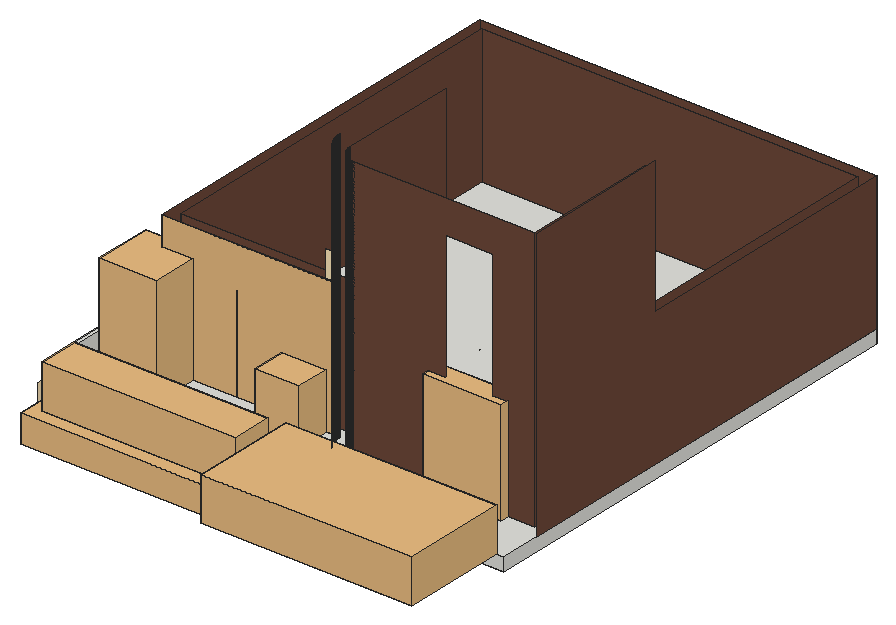
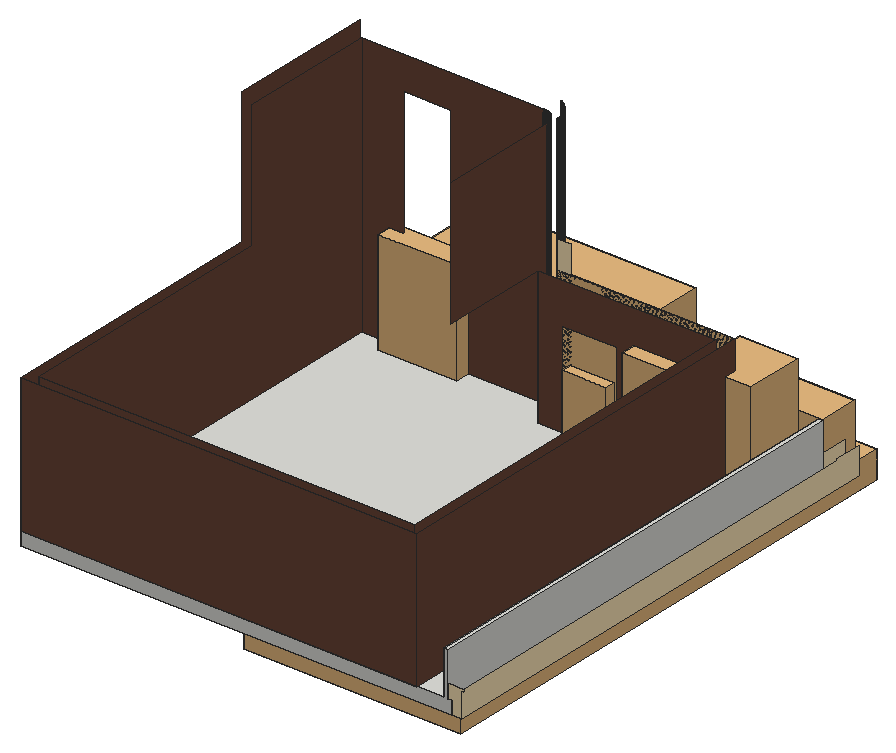
# SketchUp Ruby script. Lengths in inches.
U = 1.inch
M = Sketchup.active_model
def pt(a) = Geom::Point3d.new(a.map { |v| v * U })
def face(e, loops, mat)
  f = e.add_face(loops[0].map { |a| pt(a) })
  loops[1..].each { |l| e.add_face(l.map { |a| pt(a) }).erase! }
  f.material = f.back_material = mat if mat
  f
end
# faces: each face lists its corners as indices into pts; further lists are holes
def faces(e, pts, list, mat = nil) = list.each { |f| face(e, (f[0].is_a?(Array) ? f : [f]).map { |l| l.map { |i| pts[i] } }, mat) }
# xy, xz, yz: faces in a plane at the given z, y or x. An outline is a flat list of corners, or four numbers for a rectangle; further outlines are holes
def ring(l) = l.size == 4 ? [[l[0], l[1]], [l[2], l[1]], [l[2], l[3]], [l[0], l[3]]] : l.each_slice(2).to_a
def flat(e, list, mat, &to3) = list.each { |f| face(e, (f[0].is_a?(Array) ? f : [f]).map { |l| ring(l).map { |u, v| to3.(u, v) } }, mat) }
def xy(e, z, list, mat = nil) = flat(e, list, mat) { |x, y| [x, y, z] }
def xz(e, y, list, mat = nil) = flat(e, list, mat) { |x, z| [x, y, z] }
def yz(e, x, list, mat = nil) = flat(e, list, mat) { |y, z| [x, y, z] }
def lines(e, pts, list) = list.each { |a, b| e.add_line(pt(pts[a]), pt(pts[b])) }
# prism: a flat outline (further loops are holes) pulled along v
def prism(e, loops, v, mat = nil)
  f = face(e, loops, mat); d = Geom::Vector3d.new(v.map { |x| x * U })
  f.pushpull(f.normal.samedirection?(d) ? d.length : -d.length)
end
def box(e, o, s, mat = nil) = prism(e, [[o, [o[0] + s[0], o[1], o[2]], [o[0] + s[0], o[1] + s[1], o[2]], [o[0], o[1] + s[1], o[2]]]], [0, 0, s[2]], mat)
def at(x, y, z, deg = 0) = Geom::Transformation.translation(pt([x, y, z])) * Geom::Transformation.rotation(ORIGIN, Z_AXIS, deg.degrees)
def axes(o, x, y, z) = Geom::Transformation.new([*x, 0, *y, 0, *z, 0, *pt(o).to_a, 1])
def part(name) = M.definitions.add(name)
# library, detail: a bought-in or finely detailed component or shape, given as its bounding box
def library(name, o, s) = part(name).tap { |d| box(d.entities, o, s) }
def detail(e, o, s) = box(e.add_group.entities, o, s)
def put(e, d, t, mat = nil) = e.add_instance(d, t).tap { |i| i.material = mat if mat }
def group(e, t, mat = nil) = e.add_group.tap { |g| g.transformation = t; g.material = mat if mat }.entities
root = M.entities
M.materials.add("1026 AP 7946 SUNNY SIDE UP").color = [254, 231, 186]
M.materials.add("1916 AP K226 Macadamia Cream-N").color = [109, 72, 58]
M.materials.add("[Steel Brushed Stainless]").color = [48, 48, 48]
M.materials.add("[Wood Cherry Original]").color = [152, 86, 42]
c1 = library("Group\#76",[0,0,0],[126.13,128.06,238.18])
c2 = library("12",[-59.59,-13.96,-2.03],[132.77,19.46,130.2])
c3 = library("plant",[-35.72,-28.42,0],[66.31,67.39,84.38])
c4 = library("Group\#41",[0,-0.25,0],[156,0.25,120])
c5 = library("Glass Door",[0,0,0],[72,3.54,96])
c6 = library("Group\#22",[0,0,0],[186.93,93,38])
c7 = library("Group\#29",[0,0,0],[170,35.5,38])
c8 = library("Group\#53",[0,0,0.49],[191,455,12.72])
xy(root,132,[[15.03,254,18,674]],"1026 AP 7946 SUNNY SIDE UP")
xy(root,132,[[384,302,384,665,54,665,54,335,69,335,69,326,45,326,45,674,393,674,393,302],[224.53,302,224.29,302.01,224.06,302.02,223.82,302.03,223.59,302.04,223.35,302.06,223.12,302.07,222.88,302.09,222.65,302.12,222.41,302.14,221.95,302.2,221.71,302.23,221.48,302.26,221.25,302.3,221.01,302.33,220.55,302.42,220.32,302.46,219.86,302.56,219.625,302.61,219.4,302.66,218.71,302.84,218.49,302.9,218.26,302.97,218.03,303.03,217.81,303.1,217.58,303.17,217.36,303.25,217.14,303.32,216.91,303.4,216.69,303.48,216.47,303.57,216.25,303.65,216.03,303.74,215.82,303.83,215.38,304.01,215.17,304.11,214.95,304.2,214.74,304.3,214.53,304.41,214.31,304.51,214.1,304.62,213.89,304.72,213.6875,304.83,213.48,304.95,213.27,305.06,213.07,305.18,212.86,305.29,212.66,305.41,212.46,305.54,212.26,305.66,212.0625,305.79,211.86,305.91,211.67,306.04,211.47,306.18,211.28,306.31,211.08,306.45,210.89,306.58,210.51,306.86,210.33,307.01,210.14,307.15,209.96,307.3,209.77,307.45,209.23,307.9,209.06,308.06,208.88,308.22,208.71,308.375,208.54,308.54,208.2,308.86,207.86,309.2,207.54,309.54,207.375,309.71,207.22,309.88,207.06,310.06,206.9,310.23,206.45,310.77,206.3,310.96,206.15,311.14,206.01,311.33,205.86,311.51,205.58,311.89,205.45,312.08,205.31,312.28,205.18,312.47,205.04,312.67,204.91,312.86,204.79,313.0625,204.66,313.26,204.54,313.46,204.41,313.66,204.29,313.86,204.18,314.07,204.06,314.27,203.95,314.48,203.83,314.6875,203.72,314.89,203.62,315.1,203.51,315.31,203.41,315.53,203.3,315.74,203.2,315.95,203.11,316.17,203.01,316.38,202.83,316.82,202.74,317.03,202.65,317.25,202.57,317.47,202.48,317.69,202.4,317.91,202.32,318.14,202.25,318.36,202.17,318.58,202.1,318.81,202.03,319.03,201.97,319.26,201.9,319.49,201.84,319.71,201.66,320.4,201.61,320.625,201.56,320.86,201.46,321.32,201.42,321.55,201.33,322.01,201.3,322.25,201.26,322.48,201.23,322.71,201.2,322.95,201.14,323.41,201.12,323.65,201.09,323.88,201.07,324.12,201.06,324.35,201.04,324.59,201.03,324.82,201.02,325.06,201.01,325.29,201,325.53,201,326,111,326,111,335,210,335,210,311,224.85,311,224.85,302],[311.52,302,347.52,311],[210,311,210,325.85,210,325.71,210.01,325.56,210.01,325.41,210.02,325.26,210.03,325.12,210.05,324.82,210.06,324.68,210.07,324.53,210.09,324.38,210.1,324.24,210.14,323.94,210.16,323.8,210.18,323.65,210.21,323.51,210.23,323.36,210.26,323.22,210.29,323.07,210.35,322.79,210.38,322.64,210.41,322.5,210.45,322.36,210.49,322.21,210.52,322.07,210.5625,321.93,210.6,321.79,210.65,321.65,210.6875,321.51,210.73,321.36,210.78,321.22,210.83,321.09,210.875,320.95,210.93,320.81,211.03,320.53,211.09,320.4,211.14,320.26,211.26,319.99,211.32,319.85,211.44,319.59,211.5,319.45,211.57,319.32,211.63,319.19,211.91,318.67,211.99,318.54,212.06,318.42,212.13,318.29,212.21,318.16,212.29,318.04,212.37,317.91,212.53,317.67,212.61,317.54,212.69,317.42,212.78,317.3,212.86,317.18,212.95,317.06,213.04,316.95,213.22,316.71,213.3125,316.6,213.4,316.48,213.5,316.37,213.59,316.26,214.09,315.71,214.1875,315.6,214.29,315.5,214.39,315.39,214.5,315.29,214.6,315.1875,214.71,315.09,215.26,314.59,215.37,314.5,215.48,314.4,215.6,314.3125,215.71,314.22,215.95,314.04,216.06,313.95,216.18,313.86,216.3,313.78,216.42,313.69,216.54,313.61,216.67,313.53,216.91,313.37,217.04,313.29,217.16,313.21,217.29,313.13,217.42,313.06,217.54,312.99,217.67,312.91,218.19,312.63,218.32,312.57,218.45,312.5,218.59,312.44,218.85,312.32,218.99,312.26,219.26,312.14,219.4,312.09,219.53,312.03,219.81,311.93,219.95,311.875,220.09,311.83,220.22,311.78,220.36,311.73,220.51,311.6875,220.65,311.65,220.79,311.6,220.93,311.5625,221.07,311.52,221.21,311.49,221.36,311.45,221.5,311.41,221.64,311.38,221.79,311.35,222.07,311.29,222.22,311.26,222.36,311.23,222.51,311.21,222.65,311.18,222.8,311.16,222.94,311.14,223.24,311.1,223.38,311.09,223.53,311.07,223.68,311.06,223.82,311.05,224.12,311.03,224.26,311.02,224.41,311.01,224.56,311.01,224.71,311,224.85,311]],"1916 AP K226 Macadamia Cream-N")
xz(root,311,[[224.71,132,224.85,363],[[224.85,132,384,363],[305.52,138,347.52,333.89]]],"1916 AP K226 Macadamia Cream-N")
xz(root,311.01,[[224.41,132,224.56,363]],"1916 AP K226 Macadamia Cream-N")
xz(root,326,[[189,132,201,276]],"1026 AP 7946 SUNNY SIDE UP")
xz(root,326,[[[45,132,69,132,69,216,111,216,111,132,201,132,201,252,45,252],[141,162,189,216]]],"1916 AP K226 Macadamia Cream-N")
xz(root,335,[[[54,132,54,252,210,252,210,132,111,132,111,216,69,216,69,132],[141,162,189,216]]],"1916 AP K226 Macadamia Cream-N")
xz(root,665,[[54,132,384,252]],"1916 AP K226 Macadamia Cream-N")
xz(root,672,[[8,120,15,126]],"1026 AP 7946 SUNNY SIDE UP")
xz(root,674,[[6,120,6,142,4,142,4,144,18,144,18,132,15.03,132,15.03,126,15,126,15,120]],"1026 AP 7946 SUNNY SIDE UP")
xz(root,674,[[45,132,393,252]],"1916 AP K226 Macadamia Cream-N")
yz(root,6,[[239,120,239,144,262.9375,144,262.9375,142,674,142,674,120]],"1026 AP 7946 SUNNY SIDE UP")
yz(root,8,[[238.99,120,672,126]],"1026 AP 7946 SUNNY SIDE UP")
yz(root,15,[[672,120,674,126]],"1026 AP 7946 SUNNY SIDE UP")
yz(root,15.03,[[254,126,674,132]],"1026 AP 7946 SUNNY SIDE UP")
yz(root,18,[[239.06,132,674,144]],"1026 AP 7946 SUNNY SIDE UP")
yz(root,45,[[326,132,674,252]],"1916 AP K226 Macadamia Cream-N")
yz(root,54,[[335,132,665,252]],"1916 AP K226 Macadamia Cream-N")
yz(root,69,[[326,132,335,216]],"1916 AP K226 Macadamia Cream-N")
yz(root,111,[[326,132,335,216]],"1916 AP K226 Macadamia Cream-N")
yz(root,201,[[325.53,132,325.76,370],[325.76,132,326,370]],"1916 AP K226 Macadamia Cream-N")
yz(root,210,[[325.71,132,325.85,363],[325.85,132,335,132,335,252,431,252,431,363,325.85,363]],"1916 AP K226 Macadamia Cream-N")
yz(root,210.01,[[325.41,132,325.56,363]],"1916 AP K226 Macadamia Cream-N")
yz(root,384,[[311,132,311,363,431,363,431,252,665,252,665,132]],"1916 AP K226 Macadamia Cream-N")
yz(root,393,[[302,132,674,132,674,252,431,252,431,370,302,370]],"1916 AP K226 Macadamia Cream-N")
p = [[215.17,304.11,132],[215.17,304.11,370],[214.95,304.2,370],[214.95,304.2,132],[214.74,304.3,370],[214.74,304.3,132],
  [214.53,304.41,370],[214.53,304.41,132],[214.31,304.51,370],[214.31,304.51,132],[214.1,304.62,370],[214.1,304.62,132],
  [213.89,304.72,370],[213.89,304.72,132],[213.6875,304.83,370],[213.6875,304.83,132],[213.48,304.95,370],[213.48,304.95,132],
  [213.27,305.06,370],[213.27,305.06,132],[213.07,305.18,370],[213.07,305.18,132],[212.86,305.29,370],[212.86,305.29,132],
  [212.66,305.41,370],[212.66,305.41,132],[212.46,305.54,370],[212.46,305.54,132],[212.26,305.66,370],[212.26,305.66,132],
  [212.0625,305.79,370],[212.0625,305.79,132],[211.86,305.91,370],[211.86,305.91,132],[211.67,306.04,370],[211.67,306.04,132],
  [211.47,306.18,370],[211.47,306.18,132],[211.28,306.31,370],[211.28,306.31,132],[211.08,306.45,370],[211.08,306.45,132],
  [210.89,306.58,370],[210.89,306.58,132],[210.7,306.72,370],[210.7,306.72,132],[210.51,306.86,370],[210.51,306.86,132],
  [210.33,307.01,370],[210.33,307.01,132],[210.14,307.15,370],[210.14,307.15,132],[209.96,307.3,370],[209.96,307.3,132],
  [209.77,307.45,370],[209.77,307.45,132],[209.59,307.6,370],[209.59,307.6,132],[209.41,307.75,370],[209.41,307.75,132],
  [209.23,307.9,370],[209.23,307.9,132],[209.06,308.06,370],[209.06,308.06,132],[208.88,308.22,370],[208.88,308.22,132],
  [208.71,308.375,370],[208.71,308.375,132],[208.54,308.54,370],[208.54,308.54,132],[208.37,308.7,370],[208.37,308.7,132],
  [208.2,308.86,370],[208.2,308.86,132],[208.03,309.03,370],[208.03,309.03,132],[207.86,309.2,370],[207.86,309.2,132],
  [207.7,309.37,370],[207.7,309.37,132],[207.54,309.54,370],[207.54,309.54,132],[207.375,309.71,370],[207.375,309.71,132],
  [207.22,309.88,370],[207.22,309.88,132],[207.06,310.06,370],[207.06,310.06,132],[206.9,310.23,370],[206.9,310.23,132],
  [206.75,310.41,370],[206.75,310.41,132],[206.6,310.59,370],[206.6,310.59,132],[206.45,310.77,370],[206.45,310.77,132],
  [206.3,310.96,370],[206.3,310.96,132],[206.15,311.14,370],[206.15,311.14,132],[223.68,311.06,132],[223.68,311.06,363],
  [223.82,311.05,363],[223.82,311.05,132],[223.97,311.04,363],[223.97,311.04,132],[224.12,311.03,363],[224.12,311.03,132],
  [224.26,311.02,363],[224.26,311.02,132],[224.41,311.01,363],[224.41,311.01,132],[224.56,311.01,132],[224.56,311.01,363],
  [224.71,311,363],[224.71,311,132],[206.01,311.33,370],[206.01,311.33,132],[222.8,311.16,132],[222.8,311.16,363],
  [222.94,311.14,363],[222.94,311.14,132],[223.09,311.12,363],[223.09,311.12,132],[223.24,311.1,363],[223.24,311.1,132],
  [223.38,311.09,363],[223.38,311.09,132],[223.53,311.07,363],[223.53,311.07,132],[222.22,311.26,132],[222.22,311.26,363],
  [222.36,311.23,363],[222.36,311.23,132],[222.51,311.21,363],[222.51,311.21,132],[222.65,311.18,363],[222.65,311.18,132],
  [205.86,311.51,370],[205.86,311.51,132],[221.64,311.38,132],[221.64,311.38,363],[221.79,311.35,363],[221.79,311.35,132],
  [221.93,311.32,363],[221.93,311.32,132],[222.07,311.29,363],[222.07,311.29,132],[221.21,311.49,132],[221.21,311.49,363],
  [221.36,311.45,363],[221.36,311.45,132],[221.5,311.41,363],[221.5,311.41,132],[205.72,311.7,370],[205.72,311.7,132],
  [220.93,311.5625,132],[220.93,311.5625,363],[221.07,311.52,363],[221.07,311.52,132],[220.51,311.6875,132],[220.51,311.6875,363],
  [220.65,311.65,363],[220.65,311.65,132],[220.79,311.6,363],[220.79,311.6,132],[205.58,311.89,370],[205.58,311.89,132],
  [220.22,311.78,132],[220.22,311.78,363],[220.36,311.73,363],[220.36,311.73,132],[219.95,311.875,132],[219.95,311.875,363],
  [220.09,311.83,363],[220.09,311.83,132],[205.45,312.08,370],[205.45,312.08,132],[219.67,311.98,132],[219.67,311.98,363],
  [219.81,311.93,363],[219.81,311.93,132],[219.4,312.09,132],[219.4,312.09,363],[219.53,312.03,363],[219.53,312.03,132],
  [205.31,312.28,370],[205.31,312.28,132],[219.125,312.2,132],[219.125,312.2,363],[219.26,312.14,363],[219.26,312.14,132],
  [218.99,312.26,132],[218.99,312.26,363],[205.18,312.47,370],[205.18,312.47,132],[218.72,312.38,132],[218.72,312.38,363],
  [218.85,312.32,363],[218.85,312.32,132],[218.45,312.5,132],[218.45,312.5,363],[218.59,312.44,363],[218.59,312.44,132],
  [205.04,312.67,370],[205.04,312.67,132],[218.32,312.57,132],[218.32,312.57,363],[218.06,312.7,132],[218.06,312.7,363],
  [218.19,312.63,363],[218.19,312.63,132],[204.91,312.86,370],[204.91,312.86,132],[217.93,312.77,132],[217.93,312.77,363],
  [217.67,312.91,132],[217.67,312.91,363],[217.8,312.84,363],[217.8,312.84,132],[204.79,313.0625,370],[204.79,313.0625,132],
  [217.54,312.99,132],[217.54,312.99,363],[217.42,313.06,132],[217.42,313.06,363],[204.66,313.26,370],[204.66,313.26,132],
  [217.16,313.21,132],[217.16,313.21,363],[217.29,313.13,363],[217.29,313.13,132],[217.04,313.29,132],[217.04,313.29,363],
  [204.54,313.46,370],[204.54,313.46,132],[216.91,313.37,132],[216.91,313.37,363],[216.67,313.53,132],[216.67,313.53,363],
  [216.79,313.45,363],[216.79,313.45,132],[204.41,313.66,370],[204.41,313.66,132],[216.54,313.61,132],[216.54,313.61,363],
  [216.42,313.69,132],[216.42,313.69,363],[204.29,313.86,370],[204.29,313.86,132],[216.3,313.78,132],[216.3,313.78,363],
  [216.18,313.86,132],[216.18,313.86,363],[204.18,314.07,370],[204.18,314.07,132],[216.06,313.95,132],[216.06,313.95,363],
  [215.83,314.13,132],[215.83,314.13,363],[215.95,314.04,363],[215.95,314.04,132],[204.06,314.27,370],[204.06,314.27,132],
  [215.71,314.22,132],[215.71,314.22,363],[215.6,314.3125,132],[215.6,314.3125,363],[203.95,314.48,370],[203.95,314.48,132],
  [215.48,314.4,132],[215.48,314.4,363],[215.37,314.5,132],[215.37,314.5,363],[203.83,314.6875,370],[203.83,314.6875,132],
  [215.26,314.59,132],[215.26,314.59,363],[215.15,314.69,132],[215.15,314.69,363],[203.72,314.89,370],[203.72,314.89,132],
  [215.04,314.79,132],[215.04,314.79,363],[214.93,314.89,132],[214.93,314.89,363],[203.62,315.1,370],[203.62,315.1,132],
  [214.82,314.99,132],[214.82,314.99,363],[214.71,315.09,132],[214.71,315.09,363],[203.51,315.31,370],[203.51,315.31,132],
  [214.6,315.1875,132],[214.6,315.1875,363],[214.5,315.29,132],[214.5,315.29,363],[203.41,315.53,370],[203.41,315.53,132],
  [214.39,315.39,132],[214.39,315.39,363],[214.29,315.5,132],[214.29,315.5,363],[203.3,315.74,370],[203.3,315.74,132],
  [214.1875,315.6,132],[214.1875,315.6,363],[214.09,315.71,132],[214.09,315.71,363],[203.2,315.95,370],[203.2,315.95,132],
  [213.99,315.82,132],[213.99,315.82,363],[213.89,315.93,132],[213.89,315.93,363],[213.79,316.04,132],[213.79,316.04,363],
  [203.11,316.17,370],[203.11,316.17,132],[213.69,316.15,132],[213.69,316.15,363],[213.59,316.26,132],[213.59,316.26,363],
  [203.01,316.38,370],[203.01,316.38,132],[213.5,316.37,132],[213.5,316.37,363],[202.92,316.6,370],[202.92,316.6,132],
  [213.4,316.48,132],[213.4,316.48,363],[213.3125,316.6,132],[213.3125,316.6,363],[202.83,316.82,370],[202.83,316.82,132],
  [213.22,316.71,132],[213.22,316.71,363],[213.13,316.83,132],[213.13,316.83,363],[202.74,317.03,370],[202.74,317.03,132],
  [213.04,316.95,132],[213.04,316.95,363],[212.95,317.06,132],[212.95,317.06,363],[202.65,317.25,370],[202.65,317.25,132],
  [212.86,317.18,132],[212.86,317.18,363],[212.78,317.3,132],[212.78,317.3,363],[202.57,317.47,370],[202.57,317.47,132],
  [212.69,317.42,132],[212.69,317.42,363],[212.61,317.54,132],[212.61,317.54,363],[202.48,317.69,370],[202.48,317.69,132],
  [212.53,317.67,132],[212.53,317.67,363],[202.4,317.91,370],[202.4,317.91,132],[212.45,317.79,132],[212.45,317.79,363],
  [212.37,317.91,132],[212.37,317.91,363],[202.32,318.14,370],[202.32,318.14,132],[212.29,318.04,132],[212.29,318.04,363],
  [212.21,318.16,132],[212.21,318.16,363],[202.25,318.36,370],[202.25,318.36,132],[212.13,318.29,132],[212.13,318.29,363],
  [212.06,318.42,132],[212.06,318.42,363],[202.17,318.58,370],[202.17,318.58,132],[211.99,318.54,132],[211.99,318.54,363],
  [211.91,318.67,132],[211.91,318.67,363],[202.1,318.81,370],[202.1,318.81,132],[211.84,318.8,132],[211.84,318.8,363],
  [202.03,319.03,370],[202.03,319.03,132],[211.77,318.93,132],[211.77,318.93,363],[211.7,319.06,132],[211.7,319.06,363],
  [201.97,319.26,370],[201.97,319.26,132],[211.63,319.19,132],[211.63,319.19,363],[211.57,319.32,132],[211.57,319.32,363],
  [201.9,319.49,370],[201.9,319.49,132],[211.5,319.45,132],[211.5,319.45,363],[201.84,319.71,370],[201.84,319.71,132],
  [211.44,319.59,132],[211.44,319.59,363],[211.38,319.72,132],[211.38,319.72,363],[201.78,319.94,370],[201.78,319.94,132],
  [211.32,319.85,132],[211.32,319.85,363],[201.72,320.17,370],[201.72,320.17,132],[211.26,319.99,132],[211.26,319.99,363],
  [211.2,320.125,132],[211.2,320.125,363],[211.14,320.26,132],[211.14,320.26,363],[201.66,320.4,370],[201.66,320.4,132],
  [211.09,320.4,132],[211.09,320.4,363],[201.61,320.625,370],[201.61,320.625,132],[211.03,320.53,132],[211.03,320.53,363],
  [210.98,320.67,132],[210.98,320.67,363],[201.56,320.86,370],[201.56,320.86,132],[210.93,320.81,132],[210.93,320.81,363],
  [210.875,320.95,132],[210.875,320.95,363],[201.51,321.09,370],[201.51,321.09,132],[210.83,321.09,132],[210.83,321.09,363],
  [201.46,321.32,370],[201.46,321.32,132],[210.78,321.22,132],[210.78,321.22,363],[210.73,321.36,132],[210.73,321.36,363],
  [201.42,321.55,370],[201.42,321.55,132],[210.6875,321.51,132],[210.6875,321.51,363],[201.375,321.78,370],[201.375,321.78,132],
  [210.65,321.65,132],[210.65,321.65,363],[210.6,321.79,132],[210.6,321.79,363],[201.33,322.01,370],[201.33,322.01,132],
  [210.5625,321.93,132],[210.5625,321.93,363],[210.52,322.07,132],[210.52,322.07,363],[201.3,322.25,370],[201.3,322.25,132],
  [210.49,322.21,132],[210.49,322.21,363],[201.26,322.48,370],[201.26,322.48,132],[210.45,322.36,132],[210.45,322.36,363],
  [210.41,322.5,132],[210.41,322.5,363],[201.23,322.71,370],[201.23,322.71,132],[210.38,322.64,132],[210.38,322.64,363],
  [210.35,322.79,132],[210.35,322.79,363],[201.2,322.95,370],[201.2,322.95,132],[210.32,322.93,132],[210.32,322.93,363],
  [201.17,323.18,370],[201.17,323.18,132],[210.29,323.07,132],[210.29,323.07,363],[210.26,323.22,132],[210.26,323.22,363],
  [201.14,323.41,370],[201.14,323.41,132],[210.23,323.36,132],[210.23,323.36,363],[201.12,323.65,370],[201.12,323.65,132],
  [210.21,323.51,132],[210.21,323.51,363],[210.18,323.65,132],[210.18,323.65,363],[201.09,323.88,370],[201.09,323.88,132],
  [210.16,323.8,132],[210.16,323.8,363],[210.14,323.94,132],[210.14,323.94,363],[201.07,324.12,370],[201.07,324.12,132],
  [210.12,324.09,132],[210.12,324.09,363],[201.06,324.35,370],[201.06,324.35,132],[210.1,324.24,132],[210.1,324.24,363],
  [210.09,324.38,132],[210.09,324.38,363],[201.04,324.59,370],[201.04,324.59,132],[210.07,324.53,132],[210.07,324.53,363],
  [210.06,324.68,132],[210.06,324.68,363],[201.03,324.82,370],[201.03,324.82,132],[210.05,324.82,132],[210.05,324.82,363],
  [201.02,325.06,370],[201.02,325.06,132],[210.04,324.97,132],[210.04,324.97,363],[210.03,325.12,132],[210.03,325.12,363],
  [201.01,325.29,370],[201.01,325.29,132],[210.02,325.26,132],[210.02,325.26,363],[201,325.53,370],[201,325.53,132],
  [210.01,325.41,132],[210.01,325.41,363],[210,325.71,132],[210,325.71,363],[210.01,325.56,363],[210.01,325.56,132]]
faces(root,p,[[0,1,2,3],[3,2,4,5],[5,4,6,7],[7,6,8,9],[9,8,10,11],[11,10,12,13],[13,12,14,15],[15,14,16,17],
  [17,16,18,19],[19,18,20,21],[21,20,22,23],[23,22,24,25],[25,24,26,27],[27,26,28,29],[29,28,30,31],[31,30,32,33],
  [33,32,34,35],[35,34,36,37],[37,36,38,39],[39,38,40,41],[41,40,42,43],[43,42,44,45],[45,44,46,47],[47,46,48,49],
  [49,48,50,51],[51,50,52,53],[53,52,54,55],[55,54,56,57],[57,56,58,59],[59,58,60,61],[61,60,62,63],[63,62,64,65],
  [65,64,66,67],[67,66,68,69],[69,68,70,71],[71,70,72,73],[73,72,74,75],[75,74,76,77],[77,76,78,79],[79,78,80,81],
  [81,80,82,83],[83,82,84,85],[85,84,86,87],[87,86,88,89],[89,88,90,91],[91,90,92,93],[93,92,94,95],[95,94,96,97],
  [97,96,98,99],[100,101,102,103],[103,102,104,105],[105,104,106,107],[107,106,108,109],[109,108,110,111],[112,113,114,115],[99,98,116,117],
  [118,119,120,121],[121,120,122,123],[123,122,124,125],[125,124,126,127],[127,126,128,129],[129,128,101,100],[130,131,132,133],[133,132,134,135],
  [135,134,136,137],[137,136,119,118],[117,116,138,139],[140,141,142,143],[143,142,144,145],[145,144,146,147],[147,146,131,130],[148,149,150,151],
  [151,150,152,153],[153,152,141,140],[139,138,154,155],[156,157,158,159],[159,158,149,148],[160,161,162,163],[163,162,164,165],[165,164,157,156],
  [155,154,166,167],[168,169,170,171],[171,170,161,160],[172,173,174,175],[175,174,169,168],[167,166,176,177],[178,179,180,181],[181,180,173,172],
  [182,183,184,185],[185,184,179,178],[177,176,186,187],[188,189,190,191],[191,190,183,182],[192,193,189,188],[187,186,194,195],[196,197,198,199],
  [199,198,193,192],[200,201,202,203],[203,202,197,196],[195,194,204,205],[206,207,201,200],[208,209,210,211],[211,210,207,206],[205,204,212,213],
  [214,215,209,208],[216,217,218,219],[219,218,215,214],[213,212,220,221],[222,223,217,216],[224,225,223,222],[221,220,226,227],[228,229,230,231],
  [231,230,225,224],[232,233,229,228],[227,226,234,235],[236,237,233,232],[238,239,240,241],[241,240,237,236],[235,234,242,243],[244,245,239,238],
  [246,247,245,244],[243,242,248,249],[250,251,247,246],[252,253,251,250],[249,248,254,255],[256,257,253,252],[258,259,260,261],[261,260,257,256],
  [255,254,262,263],[264,265,259,258],[266,267,265,264],[263,262,268,269],[270,271,267,266],[272,273,271,270],[269,268,274,275],[276,277,273,272],
  [278,279,277,276],[275,274,280,281],[282,283,279,278],[284,285,283,282],[281,280,286,287],[288,289,285,284],[290,291,289,288],[287,286,292,293],
  [294,295,291,290],[296,297,295,294],[293,292,298,299],[300,301,297,296],[302,303,301,300],[299,298,304,305],[306,307,303,302],[308,309,307,306],
  [305,304,310,311],[312,313,309,308],[314,315,313,312],[316,317,315,314],[311,310,318,319],[320,321,317,316],[322,323,321,320],[319,318,324,325],
  [326,327,323,322],[325,324,328,329],[330,331,327,326],[332,333,331,330],[329,328,334,335],[336,337,333,332],[338,339,337,336],[335,334,340,341],
  [342,343,339,338],[344,345,343,342],[341,340,346,347],[348,349,345,344],[350,351,349,348],[347,346,352,353],[354,355,351,350],[356,357,355,354],
  [353,352,358,359],[360,361,357,356],[359,358,362,363],[364,365,361,360],[366,367,365,364],[363,362,368,369],[370,371,367,366],[372,373,371,370],
  [369,368,374,375],[376,377,373,372],[378,379,377,376],[375,374,380,381],[382,383,379,378],[384,385,383,382],[381,380,386,387],[388,389,385,384],
  [387,386,390,391],[392,393,389,388],[394,395,393,392],[391,390,396,397],[398,399,395,394],[400,401,399,398],[397,396,402,403],[404,405,401,400],
  [403,402,406,407],[408,409,405,404],[410,411,409,408],[407,406,412,413],[414,415,411,410],[413,412,416,417],[418,419,415,414],[420,421,419,418],
  [422,423,421,420],[417,416,424,425],[426,427,423,422],[425,424,428,429],[430,431,427,426],[432,433,431,430],[429,428,434,435],[436,437,433,432],
  [438,439,437,436],[435,434,440,441],[442,443,439,438],[441,440,444,445],[446,447,443,442],[448,449,447,446],[445,444,450,451],[452,453,449,448],
  [451,450,454,455],[456,457,453,452],[458,459,457,456],[455,454,460,461],[462,463,459,458],[464,465,463,462],[461,460,466,467],[468,469,465,464],
  [467,466,470,471],[472,473,469,468],[474,475,473,472],[471,470,476,477],[478,479,475,474],[480,481,479,478],[477,476,482,483],[484,485,481,480],
  [483,482,486,487],[488,489,485,484],[490,491,489,488],[487,486,492,493],[494,495,491,490],[493,492,496,497],[498,499,495,494],[500,501,499,498],
  [497,496,502,503],[504,505,501,500],[506,507,505,504],[503,502,508,509],[510,511,507,506],[509,508,512,513],[514,515,511,510],[516,517,515,514],
  [513,512,518,519],[520,521,517,516],[522,523,521,520],[519,518,524,525],[526,527,523,522],[525,524,528,529],[530,531,527,526],[532,533,531,530],
  [529,528,534,535],[536,537,533,532],[535,534,538,539],[540,541,537,536],[542,543,544,545]],"1916 AP K226 Macadamia Cream-N")
put(root,c1,axes([22,285.92,131.98],[0.4,0,0],[0,0.4,0],[0,0,0.4]),"1026 AP 7946 SUNNY SIDE UP")
put(root,c2,axes([321.93,317.96,132.82],[0.52,0,0],[0,1,0],[0,0,0.7]),"1026 AP 7946 SUNNY SIDE UP")
put(root,c3,axes([171.26,312.4,132],[0.58,0,0],[0,0.58,0],[0,0,0.58]))
put(root,c4,at(45,326,132),"[Wood Cherry Original]")
put(root,c5,axes([69,326,132],[0.58333,0,0],[0,1,0],[0,0,0.875]),"1026 AP 7946 SUNNY SIDE UP")
put(root,c2,axes([87.87,343.21,132.82],[0.52,0,0],[0,1,0],[0,0,0.7]),"1026 AP 7946 SUNNY SIDE UP")
g1 = group(root,at(45,254,120))
xy(g1,0,[[-30,0,-30,420,348,420,348,12,156,12,156,0]])
xy(g1,12,[[-30,0,-27.001,420],[-27.001,0,-27,9],[-27,0,-23.001,9],[-23.001,0,156,0,156,12,348,12,348,420,-23.001,420]])
xy(g1,50,[[-27.001,9,-23.001,420]])
xz(g1,0,[[-30,0,156,12]])
xz(g1,9,[[-27.001,12,-23.001,50]])
xz(g1,12,[[156,0,348,12]])
xz(g1,420,[[-30,0,-30,12,-27.001,12,-27.001,50,-23.001,50,-23.001,12,348,12,348,0]])
yz(g1,-30,[[0,0,420,12]])
yz(g1,-27.001,[[9,12,420,50]])
yz(g1,-23.001,[[9,12,420,50]])
yz(g1,156,[[0,0,12,12]])
yz(g1,348,[[12,0,420,12]])
p = [[132,-27,12],[-15,-27,12],[144,-15,12],[143.897,-16.566,12],[143.591,-18.106,12],[143.087,-19.592,12],
  [142.392,-21,12],[141.52,-22.305,12],[140.485,-23.485,12],[139.305,-24.52,12],[138,-25.392,12],[136.592,-26.087,12],
  [135.106,-26.591,12],[133.566,-26.897,12],[-16.566,-26.897,12],[-18.106,-26.591,12],[-19.592,-26.087,12],[-21,-25.392,12],
  [-22.305,-24.52,12],[-23.485,-23.485,12],[-24.52,-22.305,12],[-25.392,-21,12],[-26.087,-19.592,12],[-26.591,-18.106,12],
  [-26.897,-16.566,12],[-27,-15,12],[-27,0,12]]
lines(g1,p,[[0,1],[2,3],[3,4],[4,5],[5,6],[6,7],[7,8],[8,9],[9,10],[10,11],[11,12],[12,13],
  [13,0],[1,14],[14,15],[15,16],[16,17],[17,18],[18,19],[19,20],[20,21],[21,22],[22,23],[23,24],
  [24,25],[25,26]])
put(g1,c6,axes([156.66,-81,12],[0.98978,0,0],[0,1,0],[0,0,1]),"[Steel Brushed Stainless]")
put(g1,c7,at(-26.5,-26.5,12),"[Steel Brushed Stainless]")
put(root,c8,axes([8,217,105.91],[1,0,0],[0,1,0],[0,0,1.9]),"1026 AP 7946 SUNNY SIDE UP")
